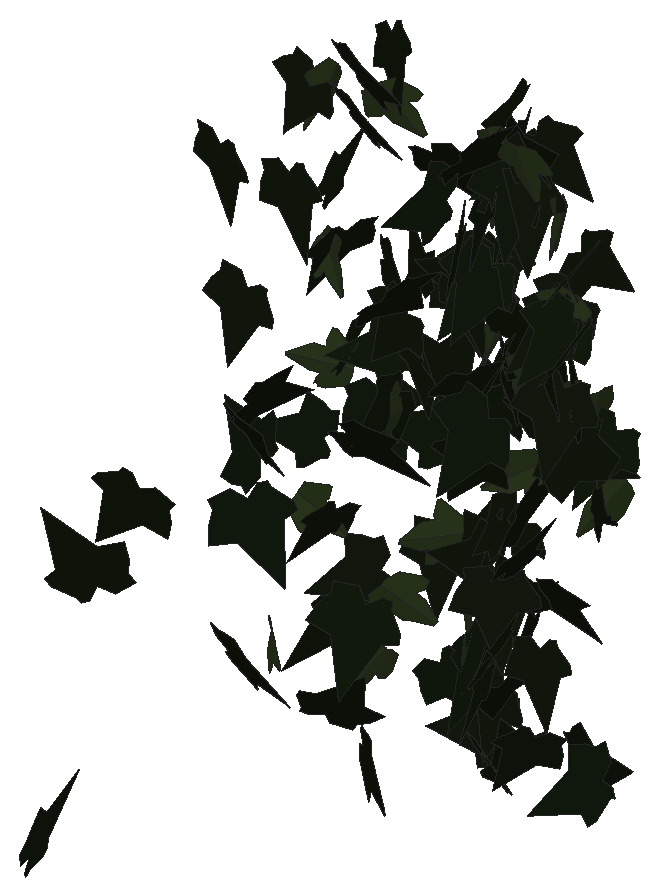
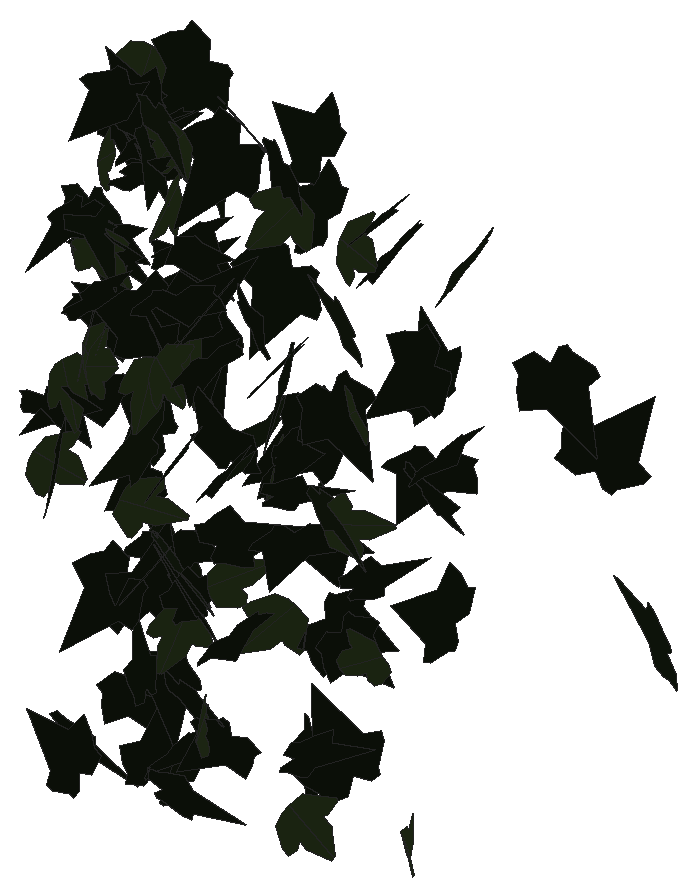
# SketchUp Ruby script. Lengths in inches.
U = 1.inch
M = Sketchup.active_model
def pt(a) = Geom::Point3d.new(a.map { |v| v * U })
def face(e, loops, mat)
  f = e.add_face(loops[0].map { |a| pt(a) })
  loops[1..].each { |l| e.add_face(l.map { |a| pt(a) }).erase! }
  f.material = f.back_material = mat if mat
  f
end
# faces: each face lists its corners as indices into pts; further lists are holes
def faces(e, pts, list, mat = nil) = list.each { |f| face(e, (f[0].is_a?(Array) ? f : [f]).map { |l| l.map { |i| pts[i] } }, mat) }
# xy, xz, yz: faces in a plane at the given z, y or x. An outline is a flat list of corners, or four numbers for a rectangle; further outlines are holes
def ring(l) = l.size == 4 ? [[l[0], l[1]], [l[2], l[1]], [l[2], l[3]], [l[0], l[3]]] : l.each_slice(2).to_a
def flat(e, list, mat, &to3) = list.each { |f| face(e, (f[0].is_a?(Array) ? f : [f]).map { |l| ring(l).map { |u, v| to3.(u, v) } }, mat) }
def xy(e, z, list, mat = nil) = flat(e, list, mat) { |x, y| [x, y, z] }
def xz(e, y, list, mat = nil) = flat(e, list, mat) { |x, z| [x, y, z] }
def yz(e, x, list, mat = nil) = flat(e, list, mat) { |y, z| [x, y, z] }
def lines(e, pts, list) = list.each { |a, b| e.add_line(pt(pts[a]), pt(pts[b])) }
# prism: a flat outline (further loops are holes) pulled along v
def prism(e, loops, v, mat = nil)
  f = face(e, loops, mat); d = Geom::Vector3d.new(v.map { |x| x * U })
  f.pushpull(f.normal.samedirection?(d) ? d.length : -d.length)
end
def box(e, o, s, mat = nil) = prism(e, [[o, [o[0] + s[0], o[1], o[2]], [o[0] + s[0], o[1] + s[1], o[2]], [o[0], o[1] + s[1], o[2]]]], [0, 0, s[2]], mat)
def at(x, y, z, deg = 0) = Geom::Transformation.translation(pt([x, y, z])) * Geom::Transformation.rotation(ORIGIN, Z_AXIS, deg.degrees)
def axes(o, x, y, z) = Geom::Transformation.new([*x, 0, *y, 0, *z, 0, *pt(o).to_a, 1])
def part(name) = M.definitions.add(name)
# library, detail: a bought-in or finely detailed component or shape, given as its bounding box
def library(name, o, s) = part(name).tap { |d| box(d.entities, o, s) }
def detail(e, o, s) = box(e.add_group.entities, o, s)
def put(e, d, t, mat = nil) = e.add_instance(d, t).tap { |i| i.material = mat if mat }
def group(e, t, mat = nil) = e.add_group.tap { |g| g.transformation = t; g.material = mat if mat }.entities
root = M.entities
M.materials.add("efeu1").color = [18, 25, 13]
M.materials.add("efeu2").color = [43, 57, 29]
c1 = part("ivyleaf_9")
p = [[1.54,2.16,1.25],[1.36,2.04,1.19],[-0.21,0.99,0.68],[-0.71,1.11,0.82],[-0.85,0.86,0.67],[-0.8,0.17,0.21],
  [-0.9,-0.01,0.1],[-0.67,-0.16,-0.02],[-0.08,-0.08,-0.05],[-0.03,-0.6,-0.4],[0.65,-0.88,-0.66],[0.83,-0.6,-0.49],
  [1.29,-0.42,-0.43],[1.8125,-0.07,-0.26],[1.21,0.44,0.15]]
faces(c1.entities,p,[[0,1,2,3,4,5,6,7,8,9,10,11,12,13,14]],"efeu1")
c2 = part("ivyleaf_10")
p = [[0,0.5,-0.03],[-0.0625,2.02,-0.43],[-0.19,2.01,-0.46],[-0.54,1.05,-0.29],[-0.52,0.625,-0.18],[-0.83,0.76,-0.28],
  [-1.16,0.64,-0.33],[-1.15,0.33,-0.24],[-0.77,-0.39,0.02],[-0.3,-0.51,0.16],[0.04,-0.48,0.23],[-0.02,2.01,-0.4375],
  [-0.06,2.01,-0.43],[0.04,-0.49,0.23],[0.67,-0.49,0.14],[1.38,0.36,-0.2],[1.375,0.51,-0.24],[0.81,0.65,-0.19],
  [0.62,0.59,-0.15],[0.6,1.09,-0.28],[0.5,1.23,-0.31]]
faces(c2.entities,p,[[0,1,2,3,4,5,6,7,8,9,10],[11,12,0,13,14,15,16,17,18,19,20]],"efeu2")
put(root,c1,axes([579.88,99.9,244.16],[-0.51848,1.33135,0.48846],[0.14555,-0.46738,1.42838],[1.41064,0.53756,0.03215]))
put(root,c1,axes([579.31,105.01,255.3],[0.63264,0.05474,1.30605],[-1.29321,0.23788,0.61645],[-0.1907,-1.43158,0.15237]))
put(root,c1,axes([580.86,106.06,259.95],[0.49982,0.4601,-1.2558],[-0.9031,-0.87272,-0.67919],[-0.98647,1.03209,-0.01449]))
put(root,c1,axes([581.88,111.39,249.87],[0.86508,-0.66857,0.9113],[0.70813,-0.57383,-1.09321],[0.88091,1.11784,-0.01614]))
put(root,c1,axes([582.46,111.78,260.79],[1.22568,-0.3407,-0.54294],[0.54662,-0.05634,1.26933],[-0.33477,-1.33937,0.08471]))
put(root,c1,axes([582.5,111.8,257.42],[-0.34389,-0.88281,-1.0429],[0.39783,0.96414,-0.94732],[1.30718,-0.52568,0.01394]))
put(root,c1,axes([587.46,113.69,253.03],[-1.02594,-0.91954,-0.43292],[0.36095,0.24538,-1.3766],[0.9501,-1.08616,0.05551]))
put(root,c1,axes([582.3125,112.25,262.18],[0.53473,0.88713,0.88336],[0.47085,0.74753,-1.03574],[-1.16001,0.71236,-0.01321]))
put(root,c1,axes([593.34,114.83,264.01],[-0.5452,-1.24172,0.59558],[-0.22952,-0.54967,-1.3561],[1.3579,-0.59146,0.00992]))
put(root,c1,axes([580.81,114.62,257.9],[-1.08451,0.06241,-0.80267],[-0.80294,0.01453,1.08601],[0.05881,1.34916,0.02543]))
put(root,c1,axes([592.875,115.52,250.95],[-0.84081,0.2738,-0.77264],[0.71705,-0.29065,-0.88331],[-0.3972,-1.10428,0.04092]))
put(root,c1,axes([584.66,116.07,251.02],[-0.22346,0.16305,-1.32385],[0.29924,-1.30195,-0.21087],[-1.29985,-0.32776,0.17905]))
put(root,c1,axes([592.11,115.43,261.7],[0.58084,0.57847,-0.99218],[-0.73216,-0.67013,-0.81932],[-0.88487,0.9342,0.02664]))
put(root,c1,axes([585.49,116.17,244.14],[0.20287,-0.22054,-1.30246],[1.31186,-0.12114,0.22485],[-0.15515,-1.31259,0.19809]))
put(root,c1,axes([594.02,115.58,256.43],[0.28709,1.13795,0.14114],[-0.0347,-0.13681,1.1736],[1.14614,-0.28918,0.00018]))
put(root,c1,axes([590.01,116.03,273.36],[-1.16888,0.67788,0.32122],[-0.2973,0.12739,-1.35069],[-0.6887,-1.2055,0.03789]))
put(root,c1,axes([576.67,117.13,270.86],[0.35547,-1.21612,0.46408],[0.14211,-0.44194,-1.26695],[1.29388,0.38264,0.01166]))
put(root,c1,axes([593.09,115.625,251.72],[-0.3115,1.11855,0.63387],[-0.1793,0.60804,-1.16108],[-1.27311,-0.35932,0.00843]))
put(root,c1,axes([584.99,115.91,259.85],[1.3991,0.20299,0.32695],[0.324,0.04395,-1.41375],[-0.20767,1.43613,-0.00294]))
put(root,c1,axes([582.88,116.88,244.82],[1.2568,0.5588,0.01046],[-0.01681,0.01206,1.37531],[0.55865,-1.25679,0.01784]))
put(root,c1,axes([580.34,117.36,270.6],[0.35936,-1.31283,-0.03189],[-0.01023,0.03026,-1.36113],[1.31318,0.3595,-0.00188]))
put(root,c1,axes([590.59,115.99,269.89],[0.00666,0.26994,1.37358],[-0.08881,1.37091,-0.26898],[-1.39704,-0.08586,0.02365]))
put(root,c1,axes([586.54,116.32,267.03],[0.51341,1.33083,0.45001],[0.07373,0.45293,-1.4236],[-1.40292,0.51083,0.08987]))
put(root,c1,axes([590.78,116.55,275.45],[0.60248,1.12768,0.73941],[0.28321,0.68597,-1.27695],[-1.3184,0.66268,0.06358]))
put(root,c2,axes([585.84,117.67,251.5625],[-0.72927,-0.46879,-0.88039],[0.79801,0.38003,-0.86339],[0.59835,-1.07819,0.07847]))
put(root,c1,axes([590.19,117.66,263.88],[0.34902,1.23479,-0.40666],[-0.16396,-0.37589,-1.28207],[-1.28965,0.38196,0.05295]))
put(root,c1,axes([591.25,118.42,253.49],[-0.64588,-0.99792,-0.6463],[0.31352,0.56652,-1.18806],[1.14685,-0.71689,-0.03919]))
put(root,c1,axes([576.5625,119.02,262.83],[-0.17848,-1.25088,0.38794],[0.00452,-0.39211,-1.26226],[1.30965,-0.16912,0.05723]))
put(root,c2,axes([592.72,118.13,275.67],[-1.1613,0.09247,-0.14215],[0.14188,-0.00898,-1.16497],[-0.09288,-1.16993,-0.00229]))
put(root,c1,axes([593.08,118.51,246.28],[0.13851,0.63063,-0.96191],[-0.24146,-0.93133,-0.64534],[-1.12457,0.27764,0.02009]))
put(root,c1,axes([590.28,118.8,272.45],[-0.71059,0.00722,-0.91749],[0.89256,-0.26338,-0.69336],[-0.21254,-1.1302,0.15572]))
put(root,c1,axes([589.99,119.32,268.43],[-0.51154,-1.18911,0.42605],[-0.10839,-0.41664,-1.29299],[1.25847,-0.51923,0.06182]))
put(root,c1,axes([593.04,118.99,250.4375],[0.06407,-1.19728,-0.16457],[-0.0302,0.16316,-1.1988],[1.20816,0.06757,-0.02124]))
put(root,c1,axes([594.28,119.13,263.875],[-1.03844,-0.75888,-0.53591],[0.43217,0.3169,-1.28618],[0.82239,-1.12478,-0.0008]))
put(root,c1,axes([594.37,119.47,267.23],[-0.8911,-0.81659,0.25515],[-0.18906,-0.17134,-1.20867],[0.83437,-0.91093,-0.00138]))
put(root,c1,axes([595.23,118.3125,266.7],[-0.54571,1.1926,0.22534],[-0.13607,0.18539,-1.31072],[-1.20605,-0.56054,0.04592]))
put(root,c1,axes([584.85,119.86,264.125],[-0.33606,-0.8834,0.86363],[-0.01651,-0.89172,-0.91856],[1.2353,-0.25224,0.22267]))
put(root,c1,axes([584.5,119.79,260.05],[0.00847,-0.3251,-1.17649],[0.66031,-0.98827,0.27784],[-1.02655,-0.63837,0.16901]))
put(root,c1,axes([590.81,119.2,264.37],[-1.02405,0.8159,-0.63929],[0.48428,-0.41793,-1.30915],[-0.91644,-1.13256,0.02255]))
put(root,c2,axes([589.69,118.86,263.41],[0.25631,-1.15549,-0.39899],[-0.09543,0.38751,-1.18355],[1.21871,0.27336,-0.00877]))
put(root,c1,axes([589.81,119.61,268.41],[-1.24736,-0.55158,-0.06751],[0.04927,0.05545,-1.36353],[0.5535,-1.24796,-0.03075]))
put(root,c1,axes([591.04,119.8,273.46],[-0.20176,-1.39197,0.02568],[-0.04105,-0.01999,-1.40601],[1.3916,-0.20241,-0.03775]))
put(root,c1,axes([582.31,119.66,275.5],[0.39619,-0.63871,1.19356],[0.84849,-0.85186,-0.7375],[1.0548,0.92514,0.14494]))
put(root,c1,axes([581.12,119.52,253.08],[-0.30245,0.60142,-0.88442],[0.10377,-0.89826,-0.64632],[-1.06449,-0.25844,0.18828]))
put(root,c1,axes([591.94,119.47,273.22],[-0.80966,-0.79475,-0.74508],[0.53407,0.51954,-1.13453],[0.94949,-0.96993,0.0028]))
put(root,c1,axes([593.83,119.69,267.24],[-1.23339,-0.16173,0.02804],[-0.02708,-0.00914,-1.24394],[0.16189,-1.23368,0.00554]))
put(root,c1,axes([589.33,119.83,243.44],[0.33831,-0.60634,0.89815],[0.54185,-0.72019,-0.6903],[0.93847,0.6344,0.07479]))
put(root,c1,axes([587.47,118.71,273.59],[1.37693,0.4873,-0.08396],[-0.07557,-0.03812,-1.46058],[-0.48867,1.37896,-0.0107]))
put(root,c2,axes([587,120.16,253.74],[-0.03914,0.24254,1.17217],[-0.1967,-1.15816,0.23308],[1.18073,-0.1849,0.07768]))
put(root,c2,axes([585.04,118.65,259.81],[0.08451,-0.44052,-1.03923],[-0.15237,1.02815,-0.44822],[1.11841,0.17336,0.01746]))
put(root,c1,axes([590.8,119,247.91],[-0.00824,1.12461,-0.17765],[0.00853,-0.17759,-1.12462],[-1.13852,-0.00947,-0.00714]))
put(root,c1,axes([590.39,120.35,262.375],[-0.16587,-0.07296,1.41238],[0.13389,-1.41648,-0.05745],[1.40791,0.12611,0.17186]))
put(root,c1,axes([579.84,120.17,256.15],[-0.45241,-0.01575,1.0083],[-0.86666,-0.55895,-0.39759],[0.51558,-0.95338,0.21644]))
put(root,c1,axes([591.34,120.01,274.32],[0.0176,-0.21691,1.21306],[0.8258,-0.8984,-0.17263],[0.91467,0.81529,0.13251]))
put(root,c1,axes([590.81,119.91,243.51],[0.4945,0.60468,0.84448],[-0.66343,-0.53575,0.77211],[0.79915,-0.81893,0.11842]))
put(root,c2,axes([593.1,120.41,271.73],[0.12573,-0.34975,1.10376],[0.70583,-0.85695,-0.35195],[0.91783,0.70692,0.11945]))
put(root,c1,axes([591.67,120.02,272.62],[-1.09374,0.15367,-0.54522],[0.54012,-0.07441,-1.10448],[-0.17073,-1.21983,-0.00131]))
put(root,c1,axes([578.95,120.73,273.53],[-0.31341,-0.98235,0.68898],[0.01698,-0.71566,-1.01265],[1.19976,-0.24649,0.19431]))
put(root,c1,axes([581.5625,120.25,273.01],[0.67173,-0.69409,0.94764],[0.70251,-0.63752,-0.96491],[0.94142,0.97099,0.04387]))
put(root,c1,axes([593.59,119.86,263.22],[0.13986,-1.03299,0.86864],[0.02558,0.87517,1.03663],[-1.34943,-0.09048,0.10968]))
put(root,c1,axes([590.6875,120.34,251.45],[0.93531,0.28135,0.78223],[-0.75276,-0.21291,0.97666],[0.35269,-1.20056,0.01012]))
put(root,c1,axes([587.58,120.42,266.625],[0.49224,-1.20241,0.03305],[0.01685,-0.02881,-1.29926],[1.20275,0.49251,0.00468]))
put(root,c1,axes([591.89,118.96,256.88],[-0.34451,0.64939,-1.09967],[-0.71708,0.84413,0.72314],[1.05678,0.78448,0.13219]))
put(root,c2,axes([576.76,120.55,244.76],[0.02845,-0.08076,1.0831],[0.94751,-0.52776,-0.06424],[0.5309,0.94624,0.05661]))
put(root,c2,axes([579.27,119.89,252.78],[0.471,0.2162,0.97025],[0.88803,0.39094,-0.5182],[-0.44669,1.00518,-0.00715]))
put(root,c1,axes([588.83,120.54,248.3],[-1.2758,-0.05865,-0.52322],[0.52228,0.03237,-1.27713],[0.06654,-1.37855,-0.00773]))
put(root,c1,axes([595.19,120.44,244.16],[-1.28132,0.20525,0.34024],[-0.33604,0.05333,-1.29765],[-0.21206,-1.32465,0.00048]))
put(root,c2,axes([593.08,121.01,262.23],[0.19758,-0.42515,1.06104],[0.47652,-0.9481,-0.46863],[1.03898,0.51569,0.01316]))
put(root,c1,axes([585.86,119.63,266],[0.19215,0.06858,1.11893],[-0.46218,1.03912,0.01568],[-1.02132,-0.45734,0.20342]))
put(root,c2,axes([593.73,120.3,267.5],[0.84481,0.18006,-0.76482],[-0.78048,0.06261,-0.84736],[-0.09074,1.13787,0.16765]))
put(root,c2,axes([593.48,120.87,262.7],[0.42182,-0.95085,0.69676],[0.4163,-0.57218,-1.03287],[1.10285,0.57966,0.12339]))
put(root,c1,axes([588.54,121.03,252.55],[-0.17308,-0.12205,1.10477],[-0.86368,-0.68899,-0.21142],[0.69961,-0.88077,0.0123]))
put(root,c1,axes([588.26,121.22,266.25],[0.02171,-0.01708,1.38171],[-1.1384,-0.78349,0.0082],[0.78323,-1.1383,-0.02637]))
put(root,c1,axes([593.96,119.53,260.74],[0.27425,-0.11233,-1.34913],[-0.08811,1.37213,-0.13216],[1.35093,0.1123,0.26527]))
put(root,c1,axes([594.26,120.31,261.96],[0.21796,-0.84489,0.75376],[0.09468,0.77851,0.84526],[-1.12829,-0.09789,0.21653]))
put(root,c1,axes([592.09,120.07,275.42],[-0.15337,-0.45833,-1.19075],[0.45743,1.09985,-0.48225],[1.1911,-0.4814,0.03188]))
put(root,c1,axes([584.36,121.24,261.625],[0.32732,-1.16137,0.69855],[0.30272,-0.63782,-1.20226],[1.32102,0.43392,0.10242]))
put(root,c1,axes([590.34,120.46,264.73],[0.33497,-0.13995,1.31842],[1.29369,-0.26313,-0.35661],[0.29018,1.33462,0.06795]))
put(root,c1,axes([593.98,120.25,269.4],[-0.51309,1.23624,-0.04847],[-0.00008,-0.05251,-1.33834],[-1.23719,-0.51269,0.02018]))
put(root,c2,axes([589.2,120.65,274.14],[-0.96767,0.15036,-0.60938],[0.58947,-0.16694,-0.97724],[-0.21559,-1.13131,0.06321]))
put(root,c1,axes([586.39,120.49,246.82],[-0.11802,-0.3116,-1.076],[0.67425,0.84426,-0.31845],[0.89457,-0.67744,0.09806]))
put(root,c2,axes([580.1,121.21,259.35],[0.1602,0.13297,1.17261],[-0.92787,-0.71703,0.20807],[0.72922,-0.94157,0.00714]))
put(root,c1,axes([588.72,121.57,245.7],[-0.14633,-1.08269,0.32411],[-0.02712,-0.32336,-1.09242],[1.12983,-0.14798,0.01575]))
put(root,c2,axes([588.82,120.61,251.45],[-0.72881,-0.74622,-0.42917],[0.32573,0.28146,-1.04254],[0.79683,-0.79758,0.03363]))
put(root,c1,axes([585.51,121.53,252.39],[-0.08402,-1.27799,0.06757],[-0.00361,-0.06748,-1.28075],[1.27977,-0.08409,0.00083]))
put(root,c1,axes([589.54,120.93,254.99],[-1.05291,0.61637,0.0026],[-0.00585,-0.00483,-1.22004],[-0.61635,-1.0529,0.00712]))
put(root,c2,axes([579.21,121.24,265.01],[0.70847,-0.17595,0.94708],[0.9302,-0.1805,-0.72937],[0.25028,1.16889,0.02993]))
put(root,c2,axes([579.06,121.74,273.24],[0.10702,-0.86346,0.89476],[0.2768,-0.85899,-0.86205],[1.21225,0.27237,0.11785]))
put(root,c2,axes([581.82,121.63,245.15],[-0.39154,-0.8846,0.70552],[-0.30235,-0.63762,-0.96726],[1.09035,-0.49447,-0.01487]))
put(root,c1,axes([579.8,120.76,268.29],[-0.4511,1.06606,0.41731],[0.16877,-0.38171,1.15755],[1.13232,0.48159,-0.00629]))
put(root,c1,axes([583.0625,120.71,265.81],[0.74972,-0.33065,-1.03128],[-0.93699,0.43093,-0.81933],[0.54307,1.19997,0.01007]))
put(root,c1,axes([590.11,121.4,248.45],[0.07022,0.81467,0.81948],[-0.16721,-0.80519,0.81479],[1.14336,-0.16778,0.06883]))
put(root,c1,axes([585.91,121.09,260.57],[-0.76934,0.40157,1.0261],[0.83789,-0.59954,0.86286],[0.7156,1.13372,0.09285]))
put(root,c1,axes([590.38,122.08,272.73],[-0.82557,-0.55631,0.63998],[-0.39949,-0.53271,-0.97839],[0.74797,-0.89853,0.18382]))
put(root,c1,axes([591.84,120.73,252.4375],[1.35377,0.2622,-0.04909],[-0.04965,-0.00181,-1.3789],[-0.26209,1.35466,0.00766]))
put(root,c2,axes([594.8,122.125,257.79],[-0.28377,-0.71139,0.96788],[-0.08064,-0.98099,-0.74467],[1.19848,-0.23444,0.17906]))
put(root,c2,axes([590.02,121.1,263.05],[-0.5264,-1.05806,-0.43899],[0.19886,0.39139,-1.18177],[1.12812,-0.5627,0.00347]))
put(root,c2,axes([586.63,122.04,247.57],[-0.02073,0.06565,1.12865],[0.78804,-0.80858,0.0615],[0.81065,0.7877,-0.03093]))
put(root,c1,axes([594.84,120.8125,258.47],[0.45599,-0.29484,-1.13077],[-0.98053,0.56379,-0.54241],[0.63572,1.08107,-0.02553]))
put(root,c1,axes([588.81,121.61,243.93],[-0.91193,0.24759,0.84965],[-0.83195,0.17617,-0.94427],[-0.30177,-1.23389,0.03567]))
put(root,c1,axes([589.72,121.1,275.51],[-0.59386,0.95216,0.26363],[-0.17373,0.20215,-1.12148],[-0.97258,-0.6175,0.03936]))
put(root,c1,axes([587.68,121.09,252.53],[-0.78912,0.96957,0.59516],[0.37573,-0.46156,1.25011],[1.07383,0.874,-0.00005]))
put(root,c2,axes([589.13,120.66,271.55],[0.19521,-0.41456,-1.18221],[-0.01654,1.19552,-0.42196],[1.25269,0.08039,0.17866]))
put(root,c1,axes([592.42,122.47,266.32],[-0.61622,-0.87674,0.64164],[-0.29425,-0.57541,-1.06884],[1.04584,-0.67848,0.07734]))
put(root,c1,axes([594.75,122.08,260.67],[-1.10924,-0.64378,-0.16904],[0.12562,0.12013,-1.28188],[0.65364,-1.1156,-0.04049]))
put(root,c1,axes([580.01,121.63,265.72],[-0.25151,1.08805,-0.78209],[0.09653,-0.77896,-1.11475],[-1.33649,-0.26102,0.06666]))
put(root,c1,axes([580.6,121.57,260.62],[-0.88471,0.77423,-0.17755],[0.1175,-0.13528,-1.17539],[-0.78559,-0.89215,0.02415]))
put(root,c2,axes([590.17,122.09,257.34],[0.3288,0.34799,-1.06473],[-0.92587,-0.54014,-0.46246],[-0.63048,0.97468,0.12386]))
put(root,c1,axes([582,121.6875,258.47],[-0.24095,-0.98827,-0.75141],[0.17269,0.73131,-1.01721],[1.22942,-0.29641,-0.00438]))
put(root,c1,axes([582.43,122.31,260.45],[-0.73802,-0.1095,0.82678],[-0.73666,-0.43203,-0.71479],[0.39102,-1.02059,0.21388]))
put(root,c2,axes([582.43,121.46,273.64],[-0.9949,-0.17353,-0.76084],[0.74462,0.15784,-1.00968],[0.23355,-1.24249,-0.022]))
put(root,c1,axes([589.69,121.64,260.26],[1.17494,-0.70007,-0.01095],[0.02228,0.05877,-1.36629],[0.6998,1.17352,0.06189]))
put(root,c1,axes([593.15,122.13,243.63],[0.24412,-0.25417,1.2546],[0.91371,-0.85991,-0.352],[0.89653,0.9456,0.01713]))
put(root,c1,axes([587.97,122,267.73],[-0.39744,-1.09986,-0.64699],[0.19232,0.61827,-1.16919],[1.26147,-0.44078,-0.02559]))
put(root,c2,axes([593.82,121.95,262.02],[-0.13527,-1.21402,0.08141],[-0.00477,-0.08138,-1.22152],[1.21673,-0.13529,0.00426]))
put(root,c1,axes([585.41,122.29,257.09],[-0.37114,-0.06817,1.16218],[-1.1485,-0.1781,-0.37722],[0.19044,-1.20693,-0.00998]))
put(root,c1,axes([585.1875,122.21,260.6],[0.26716,-1.10871,-0.01815],[-0.00096,0.01844,-1.14043],[1.10885,0.26714,0.00339]))
put(root,c1,axes([589.43,122.59,254.02],[-0.03245,-0.91861,0.56879],[0.06825,-0.56965,-0.91611],[1.07829,0.00841,0.07511]))
put(root,c1,axes([587.85,122.89,259.82],[-0.05425,-1.05962,0.85627],[0.0108,-0.85726,-1.06016],[1.36231,-0.0354,0.0425]))
put(root,c1,axes([582.2,122.22,276.16],[-0.57228,-0.08517,-1.08809],[1.08359,0.1026,-0.57794],[0.13053,-1.22512,0.02724]))
put(root,c1,axes([580.98,122.73,248.73],[-0.69878,-0.4501,0.85865],[-0.65903,-0.55574,-0.82765],[0.71102,-0.95746,0.07674]))
put(root,c2,axes([588.24,122.53,264.54],[0.00024,-1.05884,0.61478],[0.1854,-0.60766,-1.04665],[1.21026,0.0933,0.16021]))
put(root,c1,axes([590.03,121.125,273.61],[-0.5151,0.24837,-1.19726],[-1.05652,0.5636,0.57147],[0.61555,1.17521,-0.02103]))
put(root,c1,axes([586.17,122.2,265.51],[0.0989,-1.15522,-0.38831],[-0.03282,0.38692,-1.15945],[1.21829,0.1042,0.00029]))
put(root,c1,axes([593.62,121.37,269.64],[0.35246,-0.39534,-1.02793],[-0.32593,0.9935,-0.49386],[1.052,0.44026,0.19139]))
